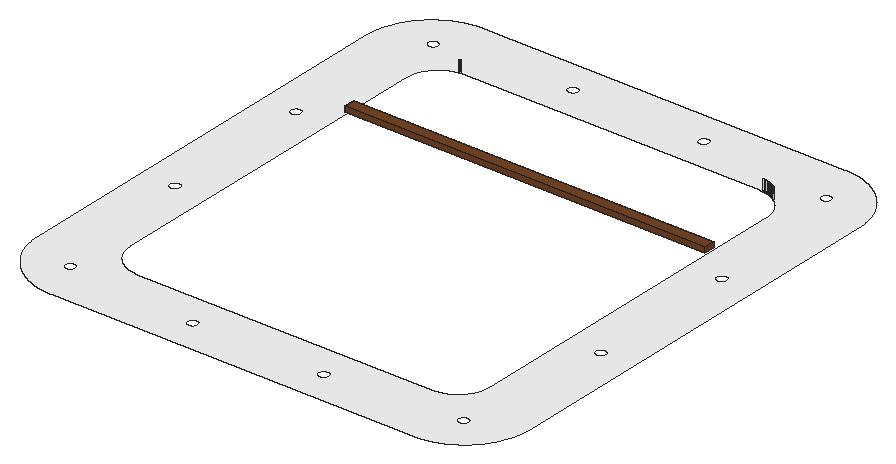
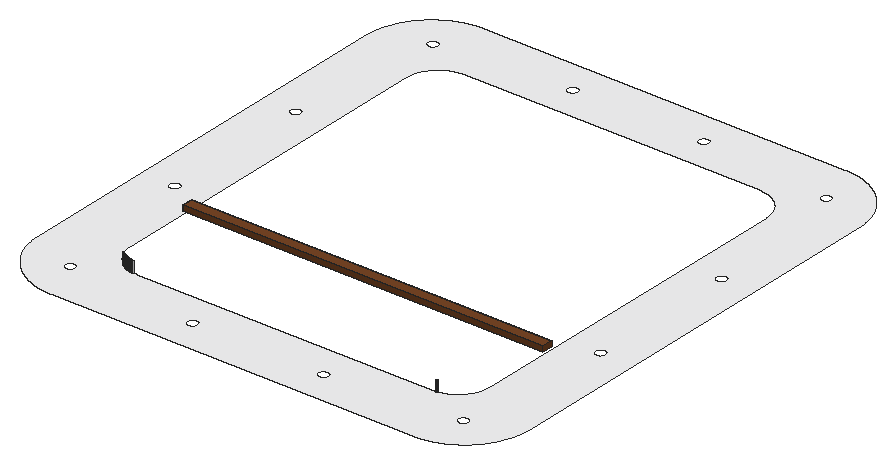
# SketchUp Ruby script. Lengths in inches.
U = 1.inch
M = Sketchup.active_model
def pt(a) = Geom::Point3d.new(a.map { |v| v * U })
def face(e, loops, mat)
  f = e.add_face(loops[0].map { |a| pt(a) })
  loops[1..].each { |l| e.add_face(l.map { |a| pt(a) }).erase! }
  f.material = f.back_material = mat if mat
  f
end
# faces: each face lists its corners as indices into pts; further lists are holes
def faces(e, pts, list, mat = nil) = list.each { |f| face(e, (f[0].is_a?(Array) ? f : [f]).map { |l| l.map { |i| pts[i] } }, mat) }
# xy, xz, yz: faces in a plane at the given z, y or x. An outline is a flat list of corners, or four numbers for a rectangle; further outlines are holes
def ring(l) = l.size == 4 ? [[l[0], l[1]], [l[2], l[1]], [l[2], l[3]], [l[0], l[3]]] : l.each_slice(2).to_a
def flat(e, list, mat, &to3) = list.each { |f| face(e, (f[0].is_a?(Array) ? f : [f]).map { |l| ring(l).map { |u, v| to3.(u, v) } }, mat) }
def xy(e, z, list, mat = nil) = flat(e, list, mat) { |x, y| [x, y, z] }
def xz(e, y, list, mat = nil) = flat(e, list, mat) { |x, z| [x, y, z] }
def yz(e, x, list, mat = nil) = flat(e, list, mat) { |y, z| [x, y, z] }
def lines(e, pts, list) = list.each { |a, b| e.add_line(pt(pts[a]), pt(pts[b])) }
# prism: a flat outline (further loops are holes) pulled along v
def prism(e, loops, v, mat = nil)
  f = face(e, loops, mat); d = Geom::Vector3d.new(v.map { |x| x * U })
  f.pushpull(f.normal.samedirection?(d) ? d.length : -d.length)
end
def box(e, o, s, mat = nil) = prism(e, [[o, [o[0] + s[0], o[1], o[2]], [o[0] + s[0], o[1] + s[1], o[2]], [o[0], o[1] + s[1], o[2]]]], [0, 0, s[2]], mat)
def at(x, y, z, deg = 0) = Geom::Transformation.translation(pt([x, y, z])) * Geom::Transformation.rotation(ORIGIN, Z_AXIS, deg.degrees)
def axes(o, x, y, z) = Geom::Transformation.new([*x, 0, *y, 0, *z, 0, *pt(o).to_a, 1])
def part(name) = M.definitions.add(name)
# library, detail: a bought-in or finely detailed component or shape, given as its bounding box
def library(name, o, s) = part(name).tap { |d| box(d.entities, o, s) }
def detail(e, o, s) = box(e.add_group.entities, o, s)
def put(e, d, t, mat = nil) = e.add_instance(d, t).tap { |i| i.material = mat if mat }
def group(e, t, mat = nil) = e.add_group.tap { |g| g.transformation = t; g.material = mat if mat }.entities
root = M.entities
M.materials.add("[Quartz Light Grey]").color = [251, 251, 252]
M.materials.add("[Wood Veneer 01]2").color = [120, 70, 37]
xy(root,111.81,[[[44.75,42,44.5,42.01,44.25,42.01,43.99,42.02,43.74,42.03,43.49,42.05,43.24,42.0625,42.99,42.08,42.74,42.11,42.49,42.13,42.24,42.16,41.99,42.1875,41.74,42.22,41.49,42.26,41.25,42.3,40.75,42.38,40.5,42.43,40.26,42.47,40.01,42.52,39.76,42.58,39.52,42.63,39.28,42.69,39.03,42.75,38.79,42.82,38.55,42.88,38.3,42.95,38.0625,43.02,37.82,43.1,37.58,43.17,37.34,43.25,37.11,43.33,36.63,43.51,36.4,43.59,36.17,43.69,35.93,43.78,35.47,43.97,35.24,44.07,35.01,44.18,34.78,44.28,34.55,44.39,34.33,44.5,34.1,44.62,33.88,44.73,33.66,44.85,33.4375,44.97,33.22,45.09,33,45.22,32.78,45.34,32.57,45.47,32.35,45.6,32.14,45.74,31.93,45.87,31.3,46.29,31.1,46.4375,30.89,46.58,30.49,46.88,30.29,47.04,30.09,47.19,29.9,47.35,29.7,47.51,29.32,47.83,29.13,48,28.94,48.16,28.75,48.33,28.57,48.5,28.39,48.68,28.21,48.85,27.85,49.21,27.68,49.39,27.5,49.57,27.33,49.75,27.16,49.94,27,50.13,26.83,50.32,26.51,50.7,26.35,50.9,26.19,51.09,26.04,51.29,25.88,51.49,25.58,51.89,25.4375,52.1,25.29,52.3,24.87,52.93,24.74,53.14,24.6,53.35,24.47,53.57,24.34,53.78,24.22,54,24.09,54.22,23.97,54.4375,23.85,54.66,23.73,54.88,23.62,55.1,23.5,55.33,23.39,55.55,23.28,55.78,23.18,56.01,23.07,56.24,22.97,56.47,22.78,56.93,22.69,57.17,22.59,57.4,22.51,57.63,22.33,58.11,22.25,58.34,22.17,58.58,22.1,58.82,22.02,59.0625,21.95,59.3,21.88,59.55,21.82,59.79,21.75,60.03,21.69,60.28,21.63,60.52,21.58,60.76,21.52,61.01,21.47,61.26,21.43,61.5,21.38,61.75,21.3,62.25,21.26,62.49,21.22,62.74,21.1875,62.99,21.16,63.24,21.13,63.49,21.11,63.74,21.08,63.99,21.0625,64.24,21.05,64.49,21.03,64.74,21.02,64.99,21.01,65.25,21.01,65.5,21,65.75,21,216.25,21.01,216.5,21.01,216.75,21.02,217.01,21.03,217.26,21.05,217.51,21.0625,217.76,21.08,218.01,21.11,218.26,21.13,218.51,21.16,218.76,21.1875,219.01,21.22,219.26,21.26,219.51,21.3,219.75,21.38,220.25,21.43,220.5,21.47,220.74,21.52,220.99,21.58,221.24,21.63,221.48,21.69,221.72,21.75,221.97,21.82,222.21,21.88,222.45,21.95,222.7,22.02,222.9375,22.1,223.18,22.17,223.42,22.25,223.66,22.33,223.89,22.51,224.37,22.59,224.6,22.69,224.83,22.78,225.07,22.97,225.53,23.07,225.76,23.18,225.99,23.28,226.22,23.39,226.45,23.5,226.67,23.62,226.9,23.73,227.12,23.85,227.34,23.97,227.5625,24.09,227.78,24.22,228,24.34,228.22,24.47,228.43,24.6,228.65,24.74,228.86,24.87,229.07,25.29,229.7,25.4375,229.9,25.58,230.11,25.88,230.51,26.04,230.71,26.19,230.91,26.35,231.1,26.51,231.3,26.83,231.68,27,231.87,27.16,232.06,27.33,232.25,27.5,232.43,27.68,232.61,27.85,232.79,28.21,233.15,28.39,233.32,28.57,233.5,28.75,233.67,28.94,233.84,29.13,234,29.32,234.17,29.7,234.49,29.9,234.65,30.09,234.81,30.29,234.96,30.49,235.12,30.89,235.42,31.1,235.5625,31.3,235.71,31.93,236.13,32.14,236.26,32.35,236.4,32.57,236.53,32.78,236.66,33,236.78,33.22,236.91,33.4375,237.03,33.66,237.15,33.88,237.27,34.1,237.38,34.33,237.5,34.55,237.61,34.78,237.72,35.01,237.82,35.24,237.93,35.47,238.03,35.93,238.22,36.17,238.31,36.4,238.41,36.63,238.49,37.11,238.67,37.34,238.75,37.58,238.83,37.82,238.9,38.0625,238.98,38.3,239.05,38.55,239.12,38.79,239.18,39.03,239.25,39.28,239.31,39.52,239.37,39.76,239.42,40.01,239.48,40.26,239.53,40.5,239.57,40.75,239.62,41.25,239.7,41.49,239.74,41.74,239.78,41.99,239.8125,42.24,239.84,42.49,239.87,42.74,239.89,42.99,239.92,43.24,239.9375,43.49,239.95,43.74,239.97,43.99,239.98,44.25,239.99,44.5,239.99,44.75,240,177.25,240,177.5,239.99,177.75,239.99,178.01,239.98,178.26,239.97,178.51,239.95,178.76,239.9375,179.01,239.92,179.26,239.89,179.51,239.87,179.76,239.84,180.01,239.8125,180.26,239.78,180.51,239.74,180.75,239.7,181.25,239.62,181.5,239.57,181.74,239.53,181.99,239.48,182.24,239.42,182.48,239.37,182.72,239.31,182.97,239.25,183.21,239.18,183.45,239.12,183.7,239.05,183.9375,238.98,184.18,238.9,184.42,238.83,184.66,238.75,184.89,238.67,185.37,238.49,185.6,238.41,185.83,238.31,186.07,238.22,186.53,238.03,186.76,237.93,186.99,237.82,187.22,237.72,187.45,237.61,187.67,237.5,187.9,237.38,188.12,237.27,188.34,237.15,188.5625,237.03,188.78,236.91,189,236.78,189.22,236.66,189.43,236.53,189.65,236.4,189.86,236.26,190.07,236.13,190.7,235.71,190.9,235.5625,191.11,235.42,191.51,235.12,191.71,234.96,191.91,234.81,192.1,234.65,192.3,234.49,192.68,234.17,192.87,234,193.06,233.84,193.25,233.67,193.43,233.5,193.61,233.32,193.79,233.15,194.15,232.79,194.32,232.61,194.5,232.43,194.67,232.25,194.84,232.06,195,231.87,195.17,231.68,195.49,231.3,195.65,231.1,195.81,230.91,195.96,230.71,196.12,230.51,196.42,230.11,196.5625,229.9,196.71,229.7,197.13,229.07,197.26,228.86,197.4,228.65,197.53,228.43,197.66,228.22,197.78,228,197.91,227.78,198.03,227.5625,198.15,227.34,198.27,227.12,198.38,226.9,198.5,226.67,198.61,226.45,198.72,226.22,198.82,225.99,198.93,225.76,199.03,225.53,199.22,225.07,199.31,224.83,199.41,224.6,199.49,224.37,199.67,223.89,199.75,223.66,199.83,223.42,199.9,223.18,199.98,222.9375,200.05,222.7,200.12,222.45,200.18,222.21,200.25,221.97,200.31,221.72,200.37,221.48,200.42,221.24,200.48,220.99,200.53,220.74,200.57,220.5,200.62,220.25,200.7,219.75,200.74,219.51,200.78,219.26,200.8125,219.01,200.84,218.76,200.87,218.51,200.89,218.26,200.92,218.01,200.9375,217.76,200.95,217.51,200.97,217.26,200.98,217.01,200.99,216.75,200.99,216.5,201,216.25,201,65.75,200.99,65.5,200.99,65.25,200.98,64.99,200.97,64.74,200.95,64.49,200.9375,64.24,200.92,63.99,200.89,63.74,200.87,63.49,200.84,63.24,200.8125,62.99,200.78,62.74,200.74,62.49,200.7,62.25,200.62,61.75,200.57,61.5,200.53,61.26,200.48,61.01,200.42,60.76,200.37,60.52,200.31,60.28,200.25,60.03,200.18,59.79,200.12,59.55,200.05,59.3,199.98,59.0625,199.9,58.82,199.83,58.58,199.75,58.34,199.67,58.11,199.49,57.63,199.41,57.4,199.31,57.17,199.22,56.93,199.03,56.47,198.93,56.24,198.82,56.01,198.72,55.78,198.61,55.55,198.5,55.33,198.38,55.1,198.27,54.88,198.15,54.66,198.03,54.4375,197.91,54.22,197.78,54,197.66,53.78,197.53,53.57,197.4,53.35,197.26,53.14,197.13,52.93,196.71,52.3,196.5625,52.1,196.42,51.89,196.12,51.49,195.96,51.29,195.81,51.09,195.65,50.9,195.49,50.7,195.17,50.32,195,50.13,194.84,49.94,194.67,49.75,194.5,49.57,194.32,49.39,194.15,49.21,193.79,48.85,193.61,48.68,193.43,48.5,193.25,48.33,193.06,48.16,192.87,48,192.68,47.83,192.3,47.51,192.1,47.35,191.91,47.19,191.71,47.04,191.51,46.88,191.11,46.58,190.9,46.4375,190.7,46.29,190.07,45.87,189.86,45.74,189.65,45.6,189.43,45.47,189.22,45.34,189,45.22,188.78,45.09,188.5625,44.97,188.34,44.85,188.12,44.73,187.9,44.62,187.67,44.5,187.45,44.39,187.22,44.28,186.99,44.18,186.76,44.07,186.53,43.97,186.07,43.78,185.83,43.69,185.6,43.59,185.37,43.51,184.89,43.33,184.66,43.25,184.42,43.17,184.18,43.1,183.9375,43.02,183.7,42.95,183.45,42.88,183.21,42.82,182.97,42.75,182.72,42.69,182.48,42.63,182.24,42.58,181.99,42.52,181.74,42.47,181.5,42.43,181.25,42.38,180.75,42.3,180.51,42.26,180.26,42.22,180.01,42.1875,179.76,42.16,179.51,42.13,179.26,42.11,179.01,42.08,178.76,42.0625,178.51,42.05,178.26,42.03,178.01,42.02,177.75,42.01,177.5,42.01,177.25,42],[56.68,66,165.3125,66,165.47,66.01,165.63,66.02,165.78,66.03,166.1,66.05,166.25,66.07,166.41,66.08,166.57,66.1,166.72,66.125,166.88,66.15,167.03,66.17,167.1875,66.2,167.34,66.23,167.49,66.26,167.65,66.3,167.8,66.33,167.95,66.37,168.11,66.41,168.41,66.49,168.86,66.64,169.01,66.6875,169.15,66.74,169.3,66.8,169.45,66.85,169.59,66.91,169.74,66.97,169.88,67.04,170.02,67.1,170.17,67.17,170.73,67.45,170.86,67.53,171,67.61,171.14,67.6875,171.27,67.77,171.4,67.85,171.54,67.9375,171.67,68.02,171.93,68.2,172.05,68.29,172.18,68.38,172.31,68.48,172.43,68.58,172.55,68.67,172.67,68.77,172.91,68.98,173.03,69.08,173.15,69.1875,173.26,69.3,173.375,69.4,173.49,69.51,173.6,69.625,173.7,69.74,173.8125,69.85,173.92,69.97,174.02,70.09,174.23,70.33,174.33,70.45,174.42,70.57,174.52,70.69,174.62,70.82,174.71,70.95,174.8,71.07,174.98,71.33,175.0625,71.46,175.15,71.6,175.23,71.73,175.3125,71.86,175.39,72,175.47,72.14,175.55,72.27,175.83,72.83,175.9,72.98,175.96,73.12,176.03,73.26,176.09,73.41,176.15,73.55,176.2,73.7,176.26,73.85,176.3125,73.99,176.36,74.14,176.51,74.59,176.59,74.89,176.63,75.05,176.67,75.2,176.7,75.35,176.74,75.51,176.77,75.66,176.8,75.8125,176.83,75.97,176.85,76.12,176.875,76.28,176.9,76.43,176.92,76.59,176.93,76.75,176.95,76.9,176.97,77.22,176.98,77.37,176.99,77.53,177,77.6875,177,204.3125,176.99,204.47,176.98,204.63,176.97,204.78,176.95,205.1,176.93,205.25,176.92,205.41,176.9,205.57,176.875,205.72,176.85,205.88,176.83,206.03,176.8,206.1875,176.77,206.34,176.74,206.49,176.7,206.65,176.67,206.8,176.63,206.95,176.59,207.11,176.51,207.41,176.36,207.86,176.3125,208.01,176.26,208.15,176.2,208.3,176.15,208.45,176.09,208.59,176.03,208.74,175.96,208.88,175.9,209.02,175.83,209.17,175.55,209.73,175.47,209.86,175.39,210,175.3125,210.14,175.23,210.27,175.15,210.4,175.0625,210.54,174.98,210.67,174.8,210.93,174.71,211.05,174.62,211.18,174.52,211.31,174.42,211.43,174.33,211.55,174.23,211.67,174.02,211.91,173.92,212.03,173.8125,212.15,173.7,212.26,173.6,212.375,173.49,212.49,173.375,212.6,173.26,212.7,173.15,212.8125,173.03,212.92,172.91,213.02,172.67,213.23,172.55,213.33,172.43,213.42,172.31,213.52,172.18,213.62,172.05,213.71,171.93,213.8,171.67,213.98,171.54,214.0625,171.4,214.15,171.27,214.23,171.14,214.3125,171,214.39,170.86,214.47,170.73,214.55,170.17,214.83,170.02,214.9,169.88,214.96,169.74,215.03,169.59,215.09,169.45,215.15,169.3,215.2,169.15,215.26,169.01,215.3125,168.86,215.36,168.41,215.51,168.11,215.59,167.95,215.63,167.8,215.67,167.65,215.7,167.49,215.74,167.34,215.77,167.1875,215.8,167.03,215.83,166.88,215.85,166.72,215.875,166.57,215.9,166.41,215.92,166.25,215.93,166.1,215.95,165.78,215.97,165.63,215.98,165.47,215.99,165.3125,216,56.6875,216,56.53,215.99,56.37,215.98,56.22,215.97,55.9,215.95,55.75,215.93,55.59,215.92,55.43,215.9,55.28,215.875,55.12,215.85,54.97,215.83,54.8125,215.8,54.66,215.77,54.51,215.74,54.35,215.7,54.2,215.67,54.05,215.63,53.89,215.59,53.59,215.51,53.14,215.36,52.99,215.3125,52.85,215.26,52.7,215.2,52.55,215.15,52.41,215.09,52.26,215.03,52.12,214.96,51.98,214.9,51.83,214.83,51.27,214.55,51.14,214.47,51,214.39,50.86,214.3125,50.73,214.23,50.6,214.15,50.46,214.0625,50.33,213.98,50.07,213.8,49.95,213.71,49.82,213.62,49.69,213.52,49.57,213.42,49.45,213.33,49.33,213.23,49.09,213.02,48.97,212.92,48.85,212.8125,48.74,212.7,48.625,212.6,48.51,212.49,48.4,212.375,48.3,212.26,48.1875,212.15,48.08,212.03,47.98,211.91,47.77,211.67,47.67,211.55,47.58,211.43,47.48,211.31,47.38,211.18,47.29,211.05,47.2,210.93,47.02,210.67,46.9375,210.54,46.85,210.4,46.77,210.27,46.6875,210.14,46.61,210,46.53,209.86,46.45,209.73,46.17,209.17,46.1,209.02,46.04,208.88,45.97,208.74,45.91,208.59,45.85,208.45,45.8,208.3,45.74,208.15,45.6875,208.01,45.64,207.86,45.49,207.41,45.41,207.11,45.37,206.95,45.33,206.8,45.3,206.65,45.26,206.49,45.23,206.34,45.2,206.1875,45.17,206.03,45.15,205.88,45.125,205.72,45.1,205.57,45.08,205.41,45.07,205.25,45.05,205.1,45.03,204.78,45.02,204.63,45.01,204.47,45,204.3125,45,77.75,45.01,77.59,45.01,77.43,45.02,77.28,45.04,76.96,45.06,76.8,45.08,76.65,45.12,76.33,45.14,76.18,45.16,76.02,45.19,75.87,45.22,75.71,45.25,75.56,45.28,75.4,45.36,75.1,45.4375,74.79,45.48,74.64,45.52,74.49,45.72,73.89,45.78,73.74,45.84,73.6,45.9,73.45,45.96,73.31,46.02,73.16,46.08,73.02,46.22,72.73,46.36,72.45,46.43,72.3125,46.51,72.17,46.59,72.04,46.75,71.76,46.91,71.5,47.36,70.85,47.46,70.72,47.55,70.6,47.65,70.48,47.75,70.35,47.85,70.23,47.96,70.11,48.06,70,48.17,69.88,48.27,69.76,48.6,69.43,48.72,69.32,48.83,69.21,48.95,69.1,49.07,69,49.19,68.89,49.55,68.59,49.67,68.5,49.8,68.4,49.93,68.31,50.05,68.21,50.18,68.125,50.3125,68.04,50.44,67.95,50.58,67.86,50.71,67.78,50.85,67.7,50.98,67.62,51.26,67.46,52.1,67.04,52.25,66.98,52.39,66.92,52.54,66.86,52.6875,66.8,52.83,66.75,52.98,66.69,53.43,66.54,53.58,66.5,53.73,66.45,53.88,66.41,54.04,66.37,54.1875,66.33,54.34,66.3,54.5,66.26,54.65,66.23,54.81,66.2,54.96,66.17,55.12,66.15,55.27,66.125,55.43,66.1,55.58,66.08,55.74,66.07,55.9,66.05,56.06,66.04,56.21,66.03,56.53,66.01],[38.9375,222.06,38.98,222.0625,39.02,222.0625,39.0625,222.06,39.1,222.07,39.1875,222.07,39.23,222.08,39.27,222.08,39.3125,222.09,39.35,222.09,39.375,222.1,39.4,222.1,39.4375,222.11,39.48,222.12,39.6,222.15,39.64,222.17,39.68,222.18,39.72,222.2,39.74,222.2,39.76,222.21,39.79,222.23,39.83,222.24,39.91,222.28,39.94,222.3,39.96,222.3125,39.98,222.32,40.02,222.34,40.05,222.36,40.09,222.39,40.16,222.43,40.19,222.46,40.23,222.48,40.29,222.54,40.32,222.5625,40.35,222.59,40.44,222.68,40.46,222.69,40.47,222.71,40.53,222.77,40.54,222.79,40.55,222.8,40.58,222.84,40.61,222.87,40.62,222.89,40.63,222.9,40.65,222.9375,40.68,222.97,40.6875,222.99,40.7,223.01,40.72,223.05,40.74,223.08,40.78,223.16,40.8,223.19,40.82,223.23,40.83,223.27,40.87,223.35,40.88,223.39,40.9,223.42,40.9,223.44,40.91,223.47,40.92,223.51,40.93,223.54,40.9375,223.57,40.94,223.59,40.95,223.625,40.96,223.67,40.96,223.6875,40.97,223.71,40.97,223.75,40.98,223.79,40.98,223.8125,40.99,223.83,40.99,223.92,41,223.9375,41,224.1875,40.99,224.21,40.99,224.29,40.98,224.3125,40.98,224.33,40.97,224.375,40.97,224.42,40.96,224.4375,40.96,224.46,40.94,224.54,40.9375,224.56,40.93,224.58,40.91,224.66,40.9,224.68,40.9,224.7,40.88,224.74,40.87,224.78,40.83,224.86,40.82,224.89,40.74,225.05,40.72,225.08,40.7,225.12,40.6875,225.13,40.68,225.15,40.65,225.1875,40.63,225.22,40.61,225.26,40.55,225.32,40.54,225.34,40.5,225.38,40.47,225.42,40.35,225.54,40.32,225.5625,40.29,225.59,40.27,225.6,40.26,225.62,40.23,225.64,40.19,225.67,40.18,225.68,40.16,225.69,40.125,225.72,40.09,225.74,40.05,225.76,40.02,225.78,39.96,225.81,39.94,225.83,39.91,225.84,39.79,225.9,39.76,225.91,39.72,225.93,39.68,225.94,39.64,225.96,39.62,225.96,39.6,225.97,39.52,225.99,39.48,226.01,39.4375,226.01,39.4,226.02,39.375,226.03,39.35,226.03,39.3125,226.04,39.27,226.04,39.25,226.05,39.1875,226.05,39.15,226.06,39.1,226.06,39.0625,226.0625,38.9375,226.0625,38.9,226.06,38.85,226.06,38.8125,226.05,38.75,226.05,38.73,226.04,38.6875,226.04,38.65,226.03,38.625,226.03,38.6,226.02,38.5625,226.01,38.52,226.01,38.48,225.99,38.4,225.97,38.38,225.96,38.36,225.96,38.32,225.94,38.28,225.93,38.24,225.91,38.21,225.9,38.09,225.84,38.06,225.83,38.04,225.81,37.98,225.78,37.95,225.76,37.91,225.74,37.875,225.72,37.84,225.69,37.82,225.68,37.81,225.67,37.77,225.64,37.74,225.62,37.73,225.6,37.71,225.59,37.68,225.5625,37.65,225.54,37.53,225.42,37.5,225.38,37.46,225.34,37.45,225.32,37.39,225.26,37.37,225.22,37.35,225.1875,37.32,225.15,37.3125,225.13,37.3,225.12,37.28,225.08,37.26,225.05,37.18,224.89,37.17,224.86,37.13,224.78,37.12,224.74,37.1,224.7,37.1,224.68,37.09,224.66,37.07,224.58,37.0625,224.56,37.06,224.54,37.04,224.46,37.04,224.4375,37.03,224.42,37.03,224.375,37.02,224.33,37.02,224.3125,37.01,224.29,37.01,224.21,37,224.1875,37,223.9375,37.01,223.92,37.01,223.83,37.02,223.8125,37.02,223.79,37.03,223.75,37.03,223.71,37.04,223.6875,37.04,223.67,37.05,223.625,37.06,223.59,37.0625,223.57,37.07,223.54,37.08,223.51,37.09,223.47,37.1,223.44,37.1,223.42,37.12,223.39,37.13,223.35,37.17,223.27,37.18,223.23,37.2,223.19,37.22,223.16,37.26,223.08,37.28,223.05,37.3,223.01,37.3125,222.99,37.32,222.97,37.35,222.9375,37.37,222.9,37.38,222.89,37.39,222.87,37.42,222.84,37.45,222.8,37.46,222.79,37.47,222.77,37.53,222.71,37.54,222.69,37.56,222.68,37.65,222.59,37.68,222.5625,37.71,222.54,37.77,222.48,37.81,222.46,37.84,222.43,37.91,222.39,37.95,222.36,37.98,222.34,38.02,222.32,38.04,222.3125,38.06,222.3,38.09,222.28,38.17,222.24,38.21,222.23,38.24,222.21,38.26,222.2,38.28,222.2,38.32,222.18,38.36,222.17,38.4,222.15,38.52,222.12,38.5625,222.11,38.6,222.1,38.625,222.1,38.65,222.09,38.6875,222.09,38.73,222.08,38.77,222.08,38.8125,222.07,38.9,222.07],[38.9,56,39.02,56,39.15,56.01,39.27,56.02,39.4,56.04,39.64,56.1,39.76,56.15,39.87,56.2,40.09,56.32,40.19,56.39,40.29,56.47,40.47,56.65,40.55,56.74,40.63,56.84,40.7,56.95,40.82,57.17,40.87,57.28,40.91,57.4,40.94,57.52,40.97,57.65,40.99,57.77,41,57.9,41,58.02,40.99,58.15,40.98,58.27,40.96,58.4,40.9,58.64,40.85,58.76,40.8,58.87,40.68,59.09,40.61,59.19,40.53,59.29,40.35,59.47,40.26,59.55,40.16,59.63,40.05,59.7,39.83,59.82,39.72,59.87,39.6,59.91,39.48,59.94,39.35,59.97,39.23,59.99,39.1,60,38.98,60,38.85,59.99,38.73,59.98,38.6,59.96,38.36,59.9,38.24,59.85,38.13,59.8,37.91,59.68,37.81,59.61,37.71,59.53,37.53,59.35,37.45,59.26,37.37,59.16,37.3,59.05,37.18,58.83,37.13,58.72,37.09,58.6,37.06,58.48,37.03,58.35,37.01,58.23,37,58.1,37,57.98,37.01,57.85,37.02,57.73,37.04,57.6,37.1,57.36,37.15,57.24,37.2,57.13,37.32,56.91,37.39,56.81,37.47,56.71,37.65,56.53,37.74,56.45,37.84,56.37,37.95,56.3,38.17,56.18,38.28,56.13,38.4,56.09,38.52,56.06,38.65,56.03,38.77,56.01],[32.9,166.71,33.15,166.71,33.27,166.73,33.4,166.75,33.52,166.78,33.64,166.8125,33.76,166.86,33.87,166.91,34.09,167.03,34.19,167.1,34.29,167.18,34.47,167.36,34.55,167.45,34.63,167.55,34.7,167.66,34.76,167.76,34.82,167.875,34.87,167.99,34.91,168.11,34.97,168.35,34.99,168.48,35,168.6,35,168.73,34.99,168.86,34.98,168.98,34.96,169.1,34.93,169.23,34.9,169.35,34.85,169.46,34.8,169.58,34.68,169.8,34.61,169.9,34.53,170,34.35,170.18,34.26,170.26,34.16,170.34,34.05,170.41,33.83,170.53,33.72,170.58,33.6,170.62,33.48,170.65,33.35,170.68,33.23,170.7,33.1,170.71,32.98,170.71,32.85,170.7,32.73,170.69,32.6,170.67,32.48,170.64,32.24,170.56,32.13,170.51,31.91,170.39,31.81,170.3125,31.71,170.24,31.62,170.15,31.53,170.0625,31.45,169.97,31.37,169.87,31.3,169.76,31.18,169.54,31.13,169.42,31.09,169.31,31.06,169.19,31.03,169.0625,31.01,168.9375,31,168.8125,31,168.6875,31.02,168.4375,31.04,168.3125,31.07,168.19,31.1,168.07,31.15,167.95,31.2,167.84,31.32,167.62,31.39,167.52,31.47,167.42,31.56,167.32,31.65,167.24,31.74,167.15,31.84,167.08,31.95,167.01,32.17,166.89,32.28,166.84,32.4,166.8,32.52,166.77,32.65,166.74,32.77,166.72],[33.02,111.35,33.15,111.36,33.27,111.37,33.4,111.39,33.52,111.42,33.76,111.5,33.87,111.55,33.98,111.61,34.09,111.68,34.19,111.75,34.29,111.83,34.38,111.91,34.47,112,34.63,112.2,34.7,112.3,34.82,112.52,34.87,112.64,34.91,112.76,34.97,113,34.99,113.125,35,113.25,35,113.375,34.98,113.625,34.96,113.75,34.9,113.99,34.8,114.23,34.74,114.34,34.68,114.44,34.61,114.55,34.53,114.65,34.35,114.83,34.26,114.91,34.16,114.98,33.94,115.12,33.72,115.22,33.48,115.3,33.35,115.32,33.23,115.34,33.1,115.35,32.85,115.35,32.73,115.34,32.6,115.31,32.48,115.29,32.24,115.21,32.13,115.15,32.02,115.1,31.91,115.03,31.81,114.96,31.71,114.88,31.62,114.8,31.53,114.71,31.37,114.51,31.3,114.41,31.24,114.3,31.18,114.1875,31.13,114.07,31.09,113.95,31.03,113.71,31.01,113.58,31,113.46,31,113.33,31.01,113.21,31.02,113.08,31.04,112.96,31.1,112.72,31.2,112.48,31.32,112.26,31.39,112.16,31.47,112.0625,31.56,111.97,31.65,111.88,31.74,111.8,31.84,111.72,31.95,111.65,32.06,111.59,32.28,111.49,32.52,111.41,32.65,111.39,32.77,111.37,32.9,111.36],[188.98,111.35,189.1,111.36,189.23,111.37,189.35,111.39,189.48,111.41,189.72,111.49,189.94,111.59,190.05,111.65,190.16,111.72,190.26,111.8,190.35,111.88,190.44,111.97,190.53,112.0625,190.61,112.16,190.68,112.26,190.8,112.48,190.9,112.72,190.96,112.96,190.98,113.08,190.99,113.21,191,113.33,191,113.46,190.99,113.58,190.97,113.71,190.91,113.95,190.87,114.07,190.82,114.1875,190.76,114.3,190.7,114.41,190.63,114.51,190.47,114.71,190.38,114.8,190.29,114.88,190.19,114.96,190.09,115.03,189.98,115.1,189.87,115.15,189.76,115.21,189.52,115.29,189.4,115.31,189.27,115.34,189.15,115.35,188.9,115.35,188.77,115.34,188.65,115.32,188.52,115.3,188.28,115.22,188.06,115.12,187.84,114.98,187.74,114.91,187.65,114.83,187.47,114.65,187.39,114.55,187.32,114.44,187.26,114.34,187.2,114.23,187.1,113.99,187.04,113.75,187.02,113.625,187,113.375,187,113.25,187.01,113.125,187.03,113,187.09,112.76,187.13,112.64,187.18,112.52,187.3,112.3,187.37,112.2,187.53,112,187.62,111.91,187.71,111.83,187.81,111.75,187.91,111.68,188.02,111.61,188.13,111.55,188.24,111.5,188.48,111.42,188.6,111.39,188.73,111.37,188.85,111.36],[182.9,56,183.02,56,183.15,56.01,183.27,56.02,183.4,56.04,183.64,56.1,183.76,56.15,183.87,56.2,184.09,56.32,184.19,56.39,184.29,56.47,184.47,56.65,184.55,56.74,184.63,56.84,184.7,56.95,184.82,57.17,184.87,57.28,184.91,57.4,184.94,57.52,184.97,57.65,184.99,57.77,185,57.9,185,58.02,184.99,58.15,184.98,58.27,184.96,58.4,184.9,58.64,184.85,58.76,184.8,58.87,184.68,59.09,184.61,59.19,184.53,59.29,184.35,59.47,184.26,59.55,184.16,59.63,184.05,59.7,183.83,59.82,183.72,59.87,183.6,59.91,183.48,59.94,183.35,59.97,183.23,59.99,183.1,60,182.98,60,182.85,59.99,182.73,59.98,182.6,59.96,182.36,59.9,182.24,59.85,182.13,59.8,181.91,59.68,181.81,59.61,181.71,59.53,181.53,59.35,181.45,59.26,181.37,59.16,181.3,59.05,181.18,58.83,181.13,58.72,181.09,58.6,181.06,58.48,181.03,58.35,181.01,58.23,181,58.1,181,57.98,181.01,57.85,181.02,57.73,181.04,57.6,181.1,57.36,181.15,57.24,181.2,57.13,181.32,56.91,181.39,56.81,181.47,56.71,181.65,56.53,181.74,56.45,181.84,56.37,181.95,56.3,182.17,56.18,182.28,56.13,182.4,56.09,182.52,56.06,182.65,56.03,182.77,56.01],[86.98,226.0625,87.1,226.07,87.23,226.08,87.35,226.09,87.48,226.12,87.6,226.15,87.72,226.2,87.83,226.24,88.05,226.36,88.16,226.43,88.26,226.51,88.35,226.59,88.53,226.77,88.61,226.87,88.68,226.97,88.8,227.19,88.85,227.31,88.9,227.42,88.93,227.54,88.96,227.67,88.98,227.79,88.99,227.92,89,228.04,89,228.17,88.99,228.29,88.97,228.42,88.91,228.66,88.87,228.78,88.82,228.89,88.76,229.01,88.7,229.12,88.63,229.22,88.47,229.42,88.38,229.51,88.29,229.59,88.19,229.67,88.09,229.74,87.87,229.86,87.76,229.91,87.64,229.96,87.4,230.02,87.27,230.04,87.15,230.06,87.02,230.0625,86.9,230.06,86.77,230.05,86.65,230.03,86.52,230.01,86.28,229.93,86.06,229.83,85.84,229.69,85.74,229.62,85.65,229.54,85.56,229.45,85.47,229.35,85.39,229.26,85.32,229.15,85.26,229.05,85.2,228.93,85.15,228.82,85.1,228.7,85.04,228.46,85.02,228.33,85.01,228.21,85,228.08,85,227.96,85.01,227.83,85.03,227.71,85.09,227.47,85.13,227.35,85.18,227.23,85.3,227.01,85.37,226.9,85.45,226.8,85.53,226.71,85.62,226.62,85.71,226.54,85.81,226.46,85.91,226.39,86.02,226.32,86.13,226.26,86.24,226.21,86.48,226.13,86.6,226.1,86.73,226.08,86.85,226.07],[182.98,222.0625,183.1,222.07,183.23,222.08,183.35,222.09,183.48,222.12,183.6,222.15,183.72,222.2,183.83,222.24,184.05,222.36,184.16,222.43,184.26,222.51,184.35,222.59,184.53,222.77,184.61,222.87,184.68,222.97,184.8,223.19,184.85,223.31,184.9,223.42,184.93,223.54,184.96,223.67,184.98,223.79,184.99,223.92,185,224.04,185,224.17,184.99,224.29,184.97,224.42,184.91,224.66,184.87,224.78,184.82,224.89,184.76,225.01,184.7,225.12,184.63,225.22,184.47,225.42,184.38,225.51,184.29,225.59,184.19,225.67,184.09,225.74,183.87,225.86,183.76,225.91,183.64,225.96,183.4,226.02,183.27,226.04,183.15,226.06,183.02,226.0625,182.9,226.06,182.77,226.05,182.65,226.03,182.52,226.01,182.28,225.93,182.06,225.83,181.84,225.69,181.74,225.62,181.65,225.54,181.56,225.45,181.47,225.35,181.39,225.26,181.32,225.15,181.26,225.05,181.2,224.93,181.15,224.82,181.1,224.7,181.04,224.46,181.02,224.33,181.01,224.21,181,224.08,181,223.96,181.01,223.83,181.03,223.71,181.09,223.47,181.13,223.35,181.18,223.23,181.3,223.01,181.37,222.9,181.45,222.8,181.53,222.71,181.62,222.62,181.71,222.54,181.81,222.46,181.91,222.39,182.02,222.32,182.13,222.26,182.24,222.21,182.48,222.13,182.6,222.1,182.73,222.08,182.85,222.07],[134.98,226.0625,135.1,226.07,135.23,226.08,135.35,226.09,135.48,226.12,135.6,226.15,135.72,226.2,135.83,226.24,136.05,226.36,136.16,226.43,136.26,226.51,136.35,226.59,136.53,226.77,136.61,226.87,136.68,226.97,136.8,227.19,136.85,227.31,136.9,227.42,136.93,227.54,136.96,227.67,136.98,227.79,136.99,227.92,137,228.04,137,228.17,136.99,228.29,136.97,228.42,136.91,228.66,136.87,228.78,136.82,228.89,136.76,229.01,136.7,229.12,136.63,229.22,136.47,229.42,136.38,229.51,136.29,229.59,136.19,229.67,136.09,229.74,135.87,229.86,135.76,229.91,135.64,229.96,135.4,230.02,135.27,230.04,135.15,230.06,135.02,230.0625,134.9,230.06,134.77,230.05,134.65,230.03,134.52,230.01,134.28,229.93,134.06,229.83,133.84,229.69,133.74,229.62,133.65,229.54,133.56,229.45,133.47,229.35,133.39,229.26,133.32,229.15,133.26,229.05,133.2,228.93,133.15,228.82,133.1,228.7,133.04,228.46,133.02,228.33,133.01,228.21,133,228.08,133,227.96,133.01,227.83,133.03,227.71,133.09,227.47,133.13,227.35,133.18,227.23,133.3,227.01,133.37,226.9,133.45,226.8,133.53,226.71,133.62,226.62,133.71,226.54,133.81,226.46,133.91,226.39,134.02,226.32,134.13,226.26,134.24,226.21,134.48,226.13,134.6,226.1,134.73,226.08,134.85,226.07],[134.9,52,135.02,52,135.15,52.01,135.27,52.02,135.4,52.04,135.64,52.1,135.76,52.15,135.87,52.2,136.09,52.32,136.19,52.39,136.29,52.47,136.47,52.65,136.55,52.74,136.63,52.84,136.7,52.95,136.82,53.17,136.87,53.28,136.91,53.4,136.94,53.52,136.97,53.65,136.99,53.77,137,53.9,137,54.02,136.99,54.15,136.98,54.27,136.96,54.4,136.9,54.64,136.85,54.76,136.8,54.87,136.68,55.09,136.61,55.19,136.53,55.29,136.35,55.47,136.26,55.55,136.16,55.63,136.05,55.7,135.83,55.82,135.72,55.87,135.6,55.91,135.48,55.94,135.35,55.97,135.23,55.99,135.1,56,134.98,56,134.85,55.99,134.73,55.98,134.6,55.96,134.36,55.9,134.24,55.85,134.13,55.8,133.91,55.68,133.81,55.61,133.71,55.53,133.53,55.35,133.45,55.26,133.37,55.16,133.3,55.05,133.18,54.83,133.13,54.72,133.09,54.6,133.06,54.48,133.03,54.35,133.01,54.23,133,54.1,133,53.98,133.01,53.85,133.02,53.73,133.04,53.6,133.1,53.36,133.15,53.24,133.2,53.13,133.32,52.91,133.39,52.81,133.47,52.71,133.65,52.53,133.74,52.45,133.84,52.37,133.95,52.3,134.17,52.18,134.28,52.13,134.4,52.09,134.52,52.06,134.65,52.03,134.77,52.01],[86.9,52,87.02,52,87.15,52.01,87.27,52.02,87.4,52.04,87.64,52.1,87.76,52.15,87.87,52.2,88.09,52.32,88.19,52.39,88.29,52.47,88.47,52.65,88.55,52.74,88.63,52.84,88.7,52.95,88.82,53.17,88.87,53.28,88.91,53.4,88.94,53.52,88.97,53.65,88.99,53.77,89,53.9,89,54.02,88.99,54.15,88.98,54.27,88.96,54.4,88.9,54.64,88.85,54.76,88.8,54.87,88.68,55.09,88.61,55.19,88.53,55.29,88.35,55.47,88.26,55.55,88.16,55.63,88.05,55.7,87.83,55.82,87.72,55.87,87.6,55.91,87.48,55.94,87.35,55.97,87.23,55.99,87.1,56,86.98,56,86.85,55.99,86.73,55.98,86.6,55.96,86.36,55.9,86.24,55.85,86.13,55.8,85.91,55.68,85.81,55.61,85.71,55.53,85.53,55.35,85.45,55.26,85.37,55.16,85.3,55.05,85.18,54.83,85.13,54.72,85.09,54.6,85.06,54.48,85.03,54.35,85.01,54.23,85,54.1,85,53.98,85.01,53.85,85.02,53.73,85.04,53.6,85.1,53.36,85.15,53.24,85.2,53.13,85.32,52.91,85.39,52.81,85.47,52.71,85.65,52.53,85.74,52.45,85.84,52.37,85.95,52.3,86.17,52.18,86.28,52.13,86.4,52.09,86.52,52.06,86.65,52.03,86.77,52.01],[188.85,166.71,189.1,166.71,189.23,166.72,189.35,166.74,189.48,166.77,189.6,166.8,189.72,166.84,189.83,166.89,190.05,167.01,190.16,167.08,190.26,167.15,190.35,167.24,190.44,167.32,190.53,167.42,190.61,167.52,190.68,167.62,190.8,167.84,190.85,167.95,190.9,168.07,190.93,168.19,190.96,168.3125,190.98,168.4375,191,168.6875,191,168.8125,190.99,168.9375,190.97,169.0625,190.94,169.19,190.91,169.31,190.87,169.42,190.82,169.54,190.7,169.76,190.63,169.87,190.55,169.97,190.47,170.0625,190.38,170.15,190.29,170.24,190.19,170.3125,190.09,170.39,189.87,170.51,189.76,170.56,189.52,170.64,189.4,170.67,189.27,170.69,189.15,170.7,189.02,170.71,188.9,170.71,188.77,170.7,188.65,170.68,188.52,170.65,188.4,170.62,188.28,170.58,188.17,170.53,187.95,170.41,187.84,170.34,187.74,170.26,187.65,170.18,187.47,170,187.39,169.9,187.32,169.8,187.2,169.58,187.15,169.46,187.1,169.35,187.07,169.23,187.04,169.1,187.02,168.98,187.01,168.86,187,168.73,187,168.6,187.01,168.48,187.03,168.35,187.09,168.11,187.13,167.99,187.18,167.875,187.24,167.76,187.3,167.66,187.37,167.55,187.45,167.45,187.53,167.36,187.71,167.18,187.81,167.1,187.91,167.03,188.13,166.91,188.24,166.86,188.36,166.8125,188.48,166.78,188.6,166.75,188.73,166.73]]],"[Quartz Light Grey]")
p = [[171.67,213.98,111.81],[171.8,213.89,111.81],[171.8,213.89,115.91],[171.67,213.98,115.91],[171.54,214.0625,111.81],[171.54,214.0625,115.91],
  [171.27,214.23,111.81],[171.4,214.15,111.81],[171.4,214.15,115.91],[171.27,214.23,115.91],[171.14,214.3125,111.81],[171.14,214.3125,115.91],
  [171,214.39,111.81],[171,214.39,115.91],[170.86,214.47,111.81],[170.86,214.47,115.91],[170.59,214.62,111.81],[170.73,214.55,111.81],
  [170.73,214.55,115.91],[170.59,214.62,115.91],[170.45,214.69,111.81],[170.45,214.69,115.91],[170.31,214.76,111.81],[170.31,214.76,115.91],
  [170.02,214.9,111.81],[170.17,214.83,111.81],[170.17,214.83,115.91],[170.02,214.9,115.91],[169.88,214.96,111.81],[169.88,214.96,115.91],
  [169.59,215.09,111.81],[169.74,215.03,111.81],[169.74,215.03,115.91],[169.59,215.09,115.91],[169.3,215.2,111.81],[169.45,215.15,111.81],
  [169.45,215.15,115.91],[169.3,215.2,115.91],[169.15,215.26,111.81],[169.15,215.26,115.91],[168.86,215.36,111.81],[169.01,215.3125,111.81],
  [169.01,215.3125,115.91],[168.86,215.36,115.91],[168.56,215.46,111.81],[168.71,215.41,111.81],[168.71,215.41,115.91],[168.56,215.46,115.91],
  [168.11,215.59,111.81],[168.26,215.55,111.81],[168.26,215.55,115.91],[168.11,215.59,115.91],[168.41,215.51,111.81],[168.41,215.51,115.91],
  [167.8,215.67,111.81],[167.95,215.63,111.81],[167.95,215.63,115.91],[167.8,215.67,115.91],[167.34,215.77,111.81],[167.49,215.74,111.81],
  [167.49,215.74,115.91],[167.34,215.77,115.91],[167.65,215.7,111.81],[167.65,215.7,115.91],[54.97,215.83,111.81],[55.12,215.85,111.81],
  [55.12,215.85,115.91],[54.97,215.83,115.91],[166.88,215.85,111.81],[167.03,215.83,111.81],[167.03,215.83,115.91],[166.88,215.85,115.91],
  [167.1875,215.8,111.81],[167.1875,215.8,115.91],[55.28,215.875,111.81],[55.28,215.875,115.91],[55.43,215.9,111.81],[55.43,215.9,115.91],
  [55.59,215.92,111.81],[55.59,215.92,115.91],[166.41,215.92,111.81],[166.57,215.9,111.81],[166.57,215.9,115.91],[166.41,215.92,115.91],
  [166.72,215.875,111.81],[166.72,215.875,115.91]]
faces(root,p,[[0,1,2,3],[4,0,3,5],[6,7,8,9],[7,4,5,8],[10,6,9,11],[12,10,11,13],[14,12,13,15],[16,17,18,19],
  [17,14,15,18],[20,16,19,21],[22,20,21,23],[24,25,26,27],[25,22,23,26],[28,24,27,29],[30,31,32,33],[31,28,29,32],
  [34,35,36,37],[35,30,33,36],[38,34,37,39],[40,41,42,43],[41,38,39,42],[44,45,46,47],[45,40,43,46],[48,49,50,51],
  [49,52,53,50],[52,44,47,53],[54,55,56,57],[55,48,51,56],[58,59,60,61],[59,62,63,60],[62,54,57,63],[64,65,66,67],
  [68,69,70,71],[69,72,73,70],[72,58,61,73],[65,74,75,66],[74,76,77,75],[76,78,79,77],[80,81,82,83],[81,84,85,82],
  [84,68,71,85]],"[Quartz Light Grey]")
g1 = group(root,at(45.18,176.07,112.83,90),"[Quartz Light Grey]")
box(g1,[0,-131.82,0],[4,131.82,1.95],"[Wood Veneer 01]2")
